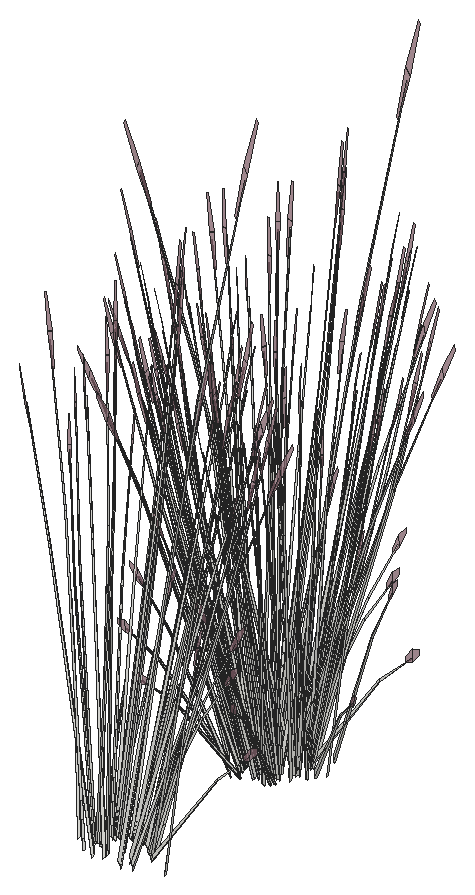
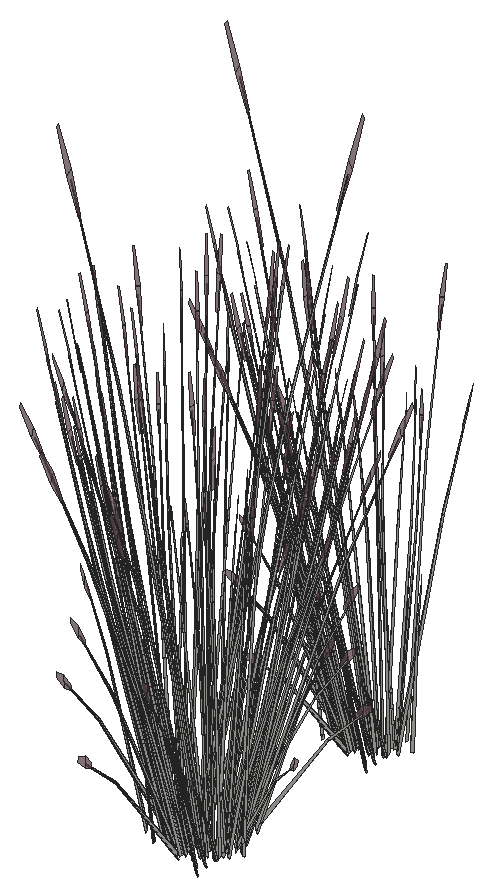
# SketchUp Ruby script. Lengths in inches.
U = 1.inch
M = Sketchup.active_model
def pt(a) = Geom::Point3d.new(a.map { |v| v * U })
def face(e, loops, mat)
  f = e.add_face(loops[0].map { |a| pt(a) })
  loops[1..].each { |l| e.add_face(l.map { |a| pt(a) }).erase! }
  f.material = f.back_material = mat if mat
  f
end
# faces: each face lists its corners as indices into pts; further lists are holes
def faces(e, pts, list, mat = nil) = list.each { |f| face(e, (f[0].is_a?(Array) ? f : [f]).map { |l| l.map { |i| pts[i] } }, mat) }
# xy, xz, yz: faces in a plane at the given z, y or x. An outline is a flat list of corners, or four numbers for a rectangle; further outlines are holes
def ring(l) = l.size == 4 ? [[l[0], l[1]], [l[2], l[1]], [l[2], l[3]], [l[0], l[3]]] : l.each_slice(2).to_a
def flat(e, list, mat, &to3) = list.each { |f| face(e, (f[0].is_a?(Array) ? f : [f]).map { |l| ring(l).map { |u, v| to3.(u, v) } }, mat) }
def xy(e, z, list, mat = nil) = flat(e, list, mat) { |x, y| [x, y, z] }
def xz(e, y, list, mat = nil) = flat(e, list, mat) { |x, z| [x, y, z] }
def yz(e, x, list, mat = nil) = flat(e, list, mat) { |y, z| [x, y, z] }
def lines(e, pts, list) = list.each { |a, b| e.add_line(pt(pts[a]), pt(pts[b])) }
# prism: a flat outline (further loops are holes) pulled along v
def prism(e, loops, v, mat = nil)
  f = face(e, loops, mat); d = Geom::Vector3d.new(v.map { |x| x * U })
  f.pushpull(f.normal.samedirection?(d) ? d.length : -d.length)
end
def box(e, o, s, mat = nil) = prism(e, [[o, [o[0] + s[0], o[1], o[2]], [o[0] + s[0], o[1] + s[1], o[2]], [o[0], o[1] + s[1], o[2]]]], [0, 0, s[2]], mat)
def at(x, y, z, deg = 0) = Geom::Transformation.translation(pt([x, y, z])) * Geom::Transformation.rotation(ORIGIN, Z_AXIS, deg.degrees)
def axes(o, x, y, z) = Geom::Transformation.new([*x, 0, *y, 0, *z, 0, *pt(o).to_a, 1])
def part(name) = M.definitions.add(name)
# library, detail: a bought-in or finely detailed component or shape, given as its bounding box
def library(name, o, s) = part(name).tap { |d| box(d.entities, o, s) }
def detail(e, o, s) = box(e.add_group.entities, o, s)
def put(e, d, t, mat = nil) = e.add_instance(d, t).tap { |i| i.material = mat if mat }
def group(e, t, mat = nil) = e.add_group.tap { |g| g.transformation = t; g.material = mat if mat }.entities
root = M.entities
M.materials.add("LightPink_Translucent").color = [144, 107, 117]
M.materials["LightPink_Translucent"].alpha = 0.75
c1 = part("blade")
p = [[2.15,0.21,22],[0,0.17,0],[0.09,0.45,0],[2.18,0.31,22],[2.29,0.31,22],[0.38,0.45,0],
  [2.48,0.24,33],[2.49,0.24,33],[2.48,0.22,33]]
faces(c1.entities,p,[[0,1,2,3],[4,5,2,3],[6,3,4,7],[8,0,3,6]])
c2 = part("seeds")
p = [[0.3,-0.1,1.38],[-0.01,-0.03,1.59],[-0.01,-0.03,0.03],[0.14,-0.07,-0.07],[0.29,-0.03,3],[0.15,0.01,3.11]]
faces(c2.entities,p,[[0,1,2,3],[1,0,4,5]],"LightPink_Translucent")
c3 = part("blade with seeds")
put(c3.entities,c1,at(0,0,0))
put(c3.entities,c2,axes([2.4,0.25,30.99],[1.5799,-0.05474,1.17369],[-0.12525,1.92788,0.29478],[-0.07173,-0.02425,1.56792]))
put(root,c3,axes([415.32,661.92,154.25],[0.20619,0.42709,-0.10273],[-0.36595,0.20988,-0.57019],[-0.15422,0.05635,0.8664]))
put(root,c3,axes([419.39,663.77,153.32],[-0.07843,-0.39649,-0.0295],[0.37072,-0.09115,-0.13375],[0.07742,0.02514,0.44114]))
put(root,c3,axes([418.43,663.76,154.25],[0.02194,-0.47967,-0.10273],[0.41546,0.01311,-0.57019],[0.16001,0.03332,0.8664]))
put(root,c3,axes([418.79,663.47,153.98],[0.08791,-0.00798,1.47793],[0.24113,-0.36643,-0.23373],[0.15637,0.04837,0.11853]))
put(root,c3,axes([415.19,663.03,154],[-0.28133,-0.19836,0.05432],[0.16379,-0.28248,0.42765],[-0.0902,0.09132,0.65209]))
put(root,c3,axes([415.32,662.51,153.27],[0.14219,-0.09977,1.44779],[0.11971,0.461,0.11706],[-0.22323,0.10419,0.61892]))
put(root,c3,axes([418.45,663.53,154.21],[0.40965,0.01136,-0.60019],[-0.02751,0.47821,0.07243],[0.17355,0.05047,0.84903]))
put(root,c3,axes([414.14,662.8,153.98],[0.0523,0.01265,1.49853],[0.16179,0.41674,-0.1416],[-0.10706,0.10938,0.26519]))
put(root,c3,axes([418.69,663.73,153.82],[0.23317,0.29531,-0.29918],[-0.26625,0.27955,0.38624],[0.13527,0.04253,0.73904]))
put(root,c3,axes([418.57,663.84,154],[-0.02064,0.35866,0.05432],[-0.3116,-0.00983,0.42765],[0.11936,0.03753,0.65209]))
put(root,c3,axes([415.23,663.2,153.82],[-0.35672,0.06741,-0.29918],[-0.09419,-0.38534,0.38624],[-0.10222,0.1035,0.73904]))
put(root,c3,axes([417.86,662.97,153.27],[-0.15222,-0.08126,1.44779],[0.31502,-0.34091,0.11706],[0.19634,0.15379,0.61892]))
put(root,c3,axes([417.88,661.9,153.78],[-0.35411,-0.24507,1.16821],[0.37391,-0.38156,0.50405],[0.11425,0.22994,1.12919]))
put(root,c3,axes([415.33,662.93,154.25],[0.37908,0.26007,-0.10273],[-0.21839,0.37663,-0.57019],[-0.1071,0.13092,0.8664]))
put(root,c3,axes([417.61,664.28,154.25],[0.2442,-0.40372,-0.10273],[0.35364,0.23259,-0.57019],[0.12293,0.11406,0.8664]))
put(root,c3,axes([415.84,662.82,153.27],[0.10236,-0.14492,1.44779],[0.25844,0.39118,0.11706],[-0.17726,0.17814,0.61892]))
put(root,c3,axes([415.52,663.24,153.95],[0.10528,0.43067,-0.43168],[-0.39868,0.07534,-0.33437],[-0.11425,0.11568,0.82598]))
put(root,c3,axes([417.29,664.62,153.98],[0.00121,-0.0571,1.49853],[0.35119,-0.25193,-0.1416],[0.12199,0.08992,0.26519]))
put(root,c3,axes([415.75,663.96,154],[-0.33677,-0.02198,0.05432],[0.00923,-0.33185,0.42765],[-0.03524,0.12712,0.65209]))
put(root,c3,axes([417.9,664.08,153.95],[0.40438,-0.11212,-0.43168],[0.07074,0.4246,-0.33437],[0.10862,0.12168,0.82598]))
put(root,c3,axes([417.7,664.43,154],[-0.18625,0.29962,0.05432],[-0.26523,-0.17444,0.42765],[0.08575,0.09606,0.65209]))
put(root,c3,axes([415.77,663.17,153.27],[0.0763,-0.16212,1.44779],[0.3201,0.3355,0.11706],[-0.1444,0.2091,0.61892]))
put(root,c3,axes([416.66,664.47,154],[-0.30197,0.1603,0.05432],[-0.1478,-0.29231,0.42765],[0.02916,0.12885,0.65209]))
put(root,c3,axes([415.85,664.09,153.82],[-0.27728,0.24833,-0.29918],[-0.26248,-0.28355,0.38624],[-0.03994,0.14407,0.73904]))
put(root,c3,axes([414.9,664.01,153.98],[-0.01019,0.09334,1.47793],[0.28908,0.3247,-0.23373],[-0.07568,0.15355,0.11853]))
put(root,c3,axes([415.82,663.8,154.56],[0.45039,0.02337,-0.11403],[-0.01231,0.44247,-0.63292],[-0.03129,0.17041,0.9617]))
put(root,c3,axes([416.66,664.3,154.25],[0.40102,-0.2196,-0.10273],[0.19707,0.38974,-0.57019],[0.05291,0.16424,0.8664]))
put(root,c3,axes([416.13,663.97,154.23],[0.29336,0.31691,-0.47917],[-0.3099,0.27755,-0.37115],[-0.04464,0.16102,0.91684]))
put(root,c3,axes([417,664.28,153.95],[0.40284,0.11824,-0.43168],[-0.13808,0.40538,-0.33437],[0.03694,0.16321,0.82598]))
put(root,c3,axes([417.23,663.44,153.27],[-0.09368,-0.15143,1.44779],[0.43286,-0.12749,0.11706],[0.09783,0.23774,0.61892]))
put(root,c3,axes([416.82,664.53,153.82],[-0.12355,0.36271,-0.29918],[-0.36044,-0.10579,0.38624],[0.03305,0.14603,0.73904]))
put(root,c3,axes([416.04,663.83,154.51],[-0.01066,0.43628,-0.66621],[-0.44902,-0.0293,0.0804],[-0.04739,0.18483,0.94242]))
put(root,c3,axes([414.87,664.97,153.98],[0.04649,-0.02848,1.49853],[0.38427,0.18941,-0.1416],[-0.00903,0.15771,0.26519]))
put(root,c3,axes([416.46,663.52,153.27],[-0.01003,-0.18103,1.44779],[0.43473,0.12009,0.11706],[-0.02689,0.25798,0.61892]))
put(root,c3,axes([416.85,664.2,154.21],[0.19559,0.38351,-0.60019],[-0.40262,0.21373,0.07243],[0.04574,0.1853,0.84903]))
put(root,c3,axes([416.5625,665.17,153.98],[0.05195,0.07595,1.47793],[0.41921,0.02984,-0.23373],[0.04216,0.1675,0.11853]))
put(root,c3,axes([415.89,664.44,152.84],[0.009,-0.24349,1.30391],[0.40497,0.12861,0.18019],[-0.03509,0.2595,0.61571]))
put(root,c3,axes([416.2,674.35,153.27],[0.09368,0.15143,1.44779],[-0.43286,0.12749,0.11706],[-0.09783,-0.23774,0.61892]))
put(root,c3,axes([416.91,673.35,153.98],[-0.06268,-0.06613,1.47793],[-0.4183,0.04193,-0.23373],[-0.06676,-0.15817,0.11853]))
put(root,c3,axes([417.35,674.47,154.21],[-0.19559,-0.38351,-0.60019],[0.40262,-0.21373,0.07243],[-0.04574,-0.1853,0.84903]))
put(root,c3,axes([418.17,674.84,154.21],[0.01066,-0.43628,-0.60019],[0.44902,0.0293,0.07243],[0.04739,-0.18483,0.84903]))
put(root,c3,axes([418.79,674.16,153.98],[-0.00396,-0.09387,1.47793],[-0.33411,-0.2713,-0.23373],[0.05166,-0.16446,0.11853]))
put(root,c3,axes([417.39,674.14,153.82],[0.12355,-0.36271,-0.29918],[0.36044,0.10579,0.38624],[-0.03305,-0.14603,0.73904]))
put(root,c3,axes([417.66,674.62,153.27],[-0.0763,0.16212,1.44779],[-0.3201,-0.3355,0.11706],[0.1444,-0.2091,0.61892]))
put(root,c3,axes([418.7,673.82,153.98],[-0.04162,0.03603,1.49853],[-0.40776,-0.12155,-0.1416],[-0.01476,-0.15722,0.26519]))
put(root,c3,axes([417.21,674.39,153.95],[-0.40284,-0.11824,-0.43168],[0.13808,-0.40538,-0.33437],[-0.03694,-0.16321,0.82598]))
put(root,c3,axes([418.08,674.7,153.95],[-0.29336,-0.31691,-0.43168],[0.3099,-0.27755,-0.33437],[0.04464,-0.16102,0.82598]))
put(root,c3,axes([416.49,673.13,153.98],[-0.00765,0.05653,1.49853],[-0.37706,0.20517,-0.1416],[-0.11096,-0.10488,0.26519]))
put(root,c3,axes([417.43,674.22,154],[0.4038,0.12331,0.40553],[-0.13808,0.40538,0.33437],[-0.02427,-0.15942,0.83914]))
put(root,c3,axes([417.55,674.37,154.25],[-0.40102,0.2196,-0.10273],[-0.19707,-0.38974,-0.57019],[-0.05291,-0.16424,0.8664]))
put(root,c3,axes([418.38,674.86,154.25],[-0.45039,-0.02337,-0.10273],[0.01231,-0.44247,-0.57019],[0.03129,-0.17041,0.8664]))
put(root,c3,axes([418.35,674.58,153.82],[0.27728,-0.24833,-0.29918],[0.26248,0.28355,0.38624],[0.03994,-0.14407,0.73904]))
put(root,c3,axes([417.54,674.19,154],[0.30197,-0.1603,0.05432],[0.1478,0.29231,0.42765],[-0.02916,-0.12885,0.65209]))
put(root,c3,axes([416.47,674.57,154.21],[-0.34944,-0.22798,-0.60019],[0.24834,-0.39949,0.07243],[-0.1266,-0.13612,0.84903]))
put(root,c3,axes([416.35,674.27,153.82],[-0.06329,-0.37991,-0.29918],[0.36182,-0.10032,0.38624],[-0.09718,-0.10887,0.73904]))
put(root,c3,axes([416.51,674.24,154],[0.18625,-0.29962,0.05432],[0.26523,0.17444,0.42765],[-0.08575,-0.09606,0.65209]))
put(root,c3,axes([415.57,674.83,153.27],[0.15222,0.08126,1.44779],[-0.31502,0.34091,0.11706],[-0.19634,-0.15379,0.61892]))
put(root,c3,axes([416.31,674.59,153.95],[-0.40438,0.11212,-0.43168],[-0.07074,-0.4246,-0.33437],[-0.10862,-0.12168,0.82598]))
put(root,c3,axes([418.35,674.67,154],[0.29182,0.32181,0.40553],[-0.3099,0.27755,0.33437],[0.05383,-0.15098,0.83914]))
put(root,c3,axes([416.59,674.21,154.59],[-0.2735,0.45217,-0.11506],[-0.39608,-0.2605,-0.63862],[-0.13768,-0.12775,0.97037]))
put(root,c3,axes([418.46,674.71,154],[0.33677,0.02198,0.05432],[-0.00923,0.33185,0.42765],[0.03524,-0.12712,0.65209]))
put(root,c3,axes([418.7,675.6,154.21],[0.21406,-0.37215,-0.60019],[0.37511,0.26448,0.07243],[0.12781,-0.13483,0.84903]))
put(root,c3,axes([418.6875,675.43,153.95],[-0.10528,-0.43067,-0.43168],[0.39868,-0.07534,-0.33437],[0.11425,-0.11568,0.82598]))
put(root,c3,axes([415.54,674.08,153.98],[-0.08817,-0.00333,1.47793],[-0.28072,0.33293,-0.23373],[-0.14978,-0.06803,0.11853]))
put(root,c3,axes([418.875,675.73,154.25],[-0.37908,-0.26007,-0.10273],[0.21839,-0.37663,-0.57019],[0.1071,-0.13092,0.8664]))
put(root,c3,axes([417.31,677.15,152.81],[0.35414,0.19019,1.27785],[-0.34693,0.40974,0.50532],[-0.1554,-0.24285,1.07126]))
put(root,c3,axes([419.81,675.62,153.98],[-0.05353,-0.00358,1.49853],[-0.22227,-0.38383,-0.1416],[0.08926,-0.1262,0.26519]))
put(root,c3,axes([418.98,675.47,153.82],[0.35672,-0.06741,-0.29918],[0.09419,0.38534,0.38624],[0.10222,-0.1035,0.73904]))
put(root,c3,axes([415.63,674.83,154],[0.02064,-0.35866,0.05432],[0.3116,0.00983,0.42765],[-0.11936,-0.03753,0.65209]))
put(root,c3,axes([415.51,674.94,153.82],[-0.23317,-0.29531,-0.29918],[0.26625,-0.27955,0.38624],[-0.13527,-0.04253,0.73904]))
put(root,c3,axes([415.76,675.14,154.21],[-0.40965,-0.01136,-0.60019],[0.02751,-0.47821,0.07243],[-0.17355,-0.05047,0.84903]))
put(root,c3,axes([419.01,675.64,154],[0.28133,0.19836,0.05432],[-0.16379,0.28248,0.42765],[0.0902,-0.09132,0.65209]))
put(root,c3,axes([420.01,676.08,153.98],[0.05687,-0.07184,1.47793],[-0.07279,-0.44069,-0.23373],[0.14268,-0.08356,0.11853]))
put(root,c3,axes([415.2,674.36,153.98],[0.03038,0.04707,1.49853],[-0.14646,0.42312,-0.1416],[-0.14833,0.00306,0.26519]))
put(root,c3,axes([415.625,675.23,153.95],[-0.29757,0.31243,-0.43168],[-0.2606,-0.33005,-0.33437],[-0.15119,-0.04754,0.82598]))
put(root,c3,axes([415.78,674.91,154.25],[-0.02194,0.47967,-0.10273],[-0.41546,-0.01311,-0.57019],[-0.16001,-0.03332,0.8664]))
put(root,c3,axes([418.89,676.75,154.25],[-0.20619,-0.42709,-0.10273],[0.36595,-0.20988,-0.57019],[0.15422,-0.05635,0.8664]))
put(root,c3,axes([418.87,676.38,153.95],[0.11102,-0.42903,-0.43168],[0.38064,0.14706,-0.33437],[0.15325,-0.03934,0.82598]))
put(root,c3,axes([415.25,675.57,153.27],[0.16998,-0.01068,1.44779],[-0.11276,0.46299,0.11706],[-0.24224,-0.02864,0.61892]))
put(root,c3,axes([418.8,676.54,154.21],[0.3601,-0.20831,-0.60019],[0.20068,0.4288,0.07243],[0.17399,-0.04871,0.84903]))
put(root,c3,axes([415.15,675.8,154],[-0.15051,-0.3216,0.05432],[0.27447,-0.15741,0.42765],[-0.12099,0.03106,0.65209]))
put(root,c3,axes([419.1,676.58,153.82],[0.34057,0.13158,-0.29918],[-0.09933,0.38387,0.38624],[0.13712,-0.0352,0.73904]))
put(root,c3,axes([415.1,675.97,153.82],[-0.34057,-0.13158,-0.29918],[0.09933,-0.38387,0.38624],[-0.13712,0.0352,0.73904]))
put(root,c3,axes([418.18,676.1,153.27],[-0.16998,0.01068,1.44779],[0.11276,-0.46299,0.11706],[0.24224,0.02864,0.61892]))
put(root,c3,axes([419.05,676.74,154],[0.15051,0.3216,0.05432],[-0.27447,0.15741,0.42765],[0.12099,-0.03106,0.65209]))
put(root,c3,axes([419.03,676.625,154],[-0.11578,0.43006,0.40553],[-0.38064,-0.14706,0.33437],[0.14969,-0.02584,0.83914]))
put(root,c3,axes([416.14,675.9,152.82],[0.11649,-0.06823,1.49584],[0.04017,0.47639,0.11706],[-0.25231,0.06321,0.53462]))
put(root,c3,axes([419.71,678.02,153.98],[-0.03706,-0.04129,1.49853],[0.08106,-0.44261,-0.1416],[0.14596,-0.02828,0.26519]))
put(root,c3,axes([414.89,676.22,153.98],[-0.06692,0.06124,1.47793],[0.00569,0.44742,-0.23373],[-0.15339,0.05818,0.11853]))
put(root,c3,axes([415.34,676.16,153.95],[-0.11102,0.42903,-0.43168],[-0.38064,-0.14706,-0.33437],[-0.15325,0.03934,0.82598]))
put(root,c3,axes([415.32,675.79,154.25],[0.20619,0.42709,-0.10273],[-0.36595,0.20988,-0.57019],[-0.15422,0.05635,0.8664]))
put(root,c3,axes([419.39,677.65,153.32],[-0.07843,-0.39649,-0.0295],[0.37072,-0.09115,-0.13375],[0.07742,0.02514,0.44114]))
put(root,c3,axes([418.43,677.64,154.25],[0.02194,-0.47967,-0.10273],[0.41546,0.01311,-0.57019],[0.16001,0.03332,0.8664]))
put(root,c3,axes([418.79,677.35,153.98],[0.08791,-0.00798,1.47793],[0.24113,-0.36643,-0.23373],[0.15637,0.04837,0.11853]))
put(root,c3,axes([415.27,676.99,154],[-0.10163,-0.43409,0.40553],[0.39868,-0.07534,0.33437],[-0.1175,0.10209,0.83914]))
put(root,c3,axes([415.19,676.91,154],[-0.28133,-0.19836,0.05432],[0.16379,-0.28248,0.42765],[-0.0902,0.09132,0.65209]))
put(root,c3,axes([415.32,676.38,153.27],[0.14219,-0.09977,1.44779],[0.11971,0.461,0.11706],[-0.22323,0.10419,0.61892]))
put(root,c3,axes([418.45,677.41,154.21],[0.40965,0.01136,-0.60019],[-0.02751,0.47821,0.07243],[0.17355,0.05047,0.84903]))
put(root,c3,axes([414.14,676.67,153.98],[0.0523,0.01265,1.49853],[0.16179,0.41674,-0.1416],[-0.10706,0.10938,0.26519]))
put(root,c3,axes([418.69,677.6,153.82],[0.23317,0.29531,-0.29918],[-0.26625,0.27955,0.38624],[0.13527,0.04253,0.73904]))
put(root,c3,axes([418.57,677.72,154],[-0.02064,0.35866,0.05432],[-0.3116,-0.00983,0.42765],[0.11936,0.03753,0.65209]))
put(root,c3,axes([415.23,677.07,153.82],[-0.35672,0.06741,-0.29918],[-0.09419,-0.38534,0.38624],[-0.10222,0.1035,0.73904]))
put(root,c3,axes([418.6,677.6,154],[-0.30217,0.31079,0.40553],[-0.2606,-0.33005,0.33437],[0.14177,0.05733,0.83914]))
put(root,c3,axes([417.86,676.85,153.27],[-0.15222,-0.08126,1.44779],[0.31502,-0.34091,0.11706],[0.19634,0.15379,0.61892]))
put(root,c3,axes([417.88,675.78,153.78],[-0.35411,-0.24507,1.16821],[0.37391,-0.38156,0.50405],[0.11425,0.22994,1.12919]))
put(root,c3,axes([415.33,676.81,154.25],[0.37908,0.26007,-0.10273],[-0.21839,0.37663,-0.57019],[-0.1071,0.13092,0.8664]))
put(root,c3,axes([417.61,678.16,154.25],[0.2442,-0.40372,-0.10273],[0.35364,0.23259,-0.57019],[0.12293,0.11406,0.8664]))
put(root,c3,axes([415.84,676.69,153.27],[0.10236,-0.14492,1.44779],[0.25844,0.39118,0.11706],[-0.17726,0.17814,0.61892]))
put(root,c3,axes([415.52,677.12,153.95],[0.10528,0.43067,-0.43168],[-0.39868,0.07534,-0.33437],[-0.11425,0.11568,0.82598]))
put(root,c3,axes([417.29,678.49,153.98],[0.00121,-0.0571,1.49853],[0.35119,-0.25193,-0.1416],[0.12199,0.08992,0.26519]))
put(root,c3,axes([415.75,677.84,154],[-0.33677,-0.02198,0.05432],[0.00923,-0.33185,0.42765],[-0.03524,0.12712,0.65209]))
put(root,c3,axes([415.85,677.87,154],[-0.29182,-0.32181,0.40553],[0.3099,-0.27755,0.33437],[-0.05383,0.15098,0.83914]))
put(root,c3,axes([417.9,677.96,153.95],[0.40438,-0.11212,-0.43168],[0.07074,0.4246,-0.33437],[0.10862,0.12168,0.82598]))
put(root,c3,axes([417.7,678.31,154],[-0.18625,0.29962,0.05432],[-0.26523,-0.17444,0.42765],[0.08575,0.09606,0.65209]))
put(root,c3,axes([415.77,677.05,153.27],[0.0763,-0.16212,1.44779],[0.3201,0.3355,0.11706],[-0.1444,0.2091,0.61892]))
put(root,c3,axes([416.66,678.35,154],[-0.30197,0.1603,0.05432],[-0.1478,-0.29231,0.42765],[0.02916,0.12885,0.65209]))
put(root,c3,axes([415.85,677.96,153.82],[-0.27728,0.24833,-0.29918],[-0.26248,-0.28355,0.38624],[-0.03994,0.14407,0.73904]))
put(root,c3,axes([414.9,677.89,153.98],[-0.01019,0.09334,1.47793],[0.28908,0.3247,-0.23373],[-0.07568,0.15355,0.11853]))
put(root,c3,axes([415.82,677.68,154.56],[0.45039,0.02337,-0.11403],[-0.01231,0.44247,-0.63292],[-0.03129,0.17041,0.9617]))
put(root,c3,axes([416.66,678.17,154.25],[0.40102,-0.2196,-0.10273],[0.19707,0.38974,-0.57019],[0.05291,0.16424,0.8664]))
put(root,c3,axes([416.13,677.85,154.23],[0.29336,0.31691,-0.47917],[-0.3099,0.27755,-0.37115],[-0.04464,0.16102,0.91684]))
put(root,c3,axes([417,678.15,153.95],[0.40284,0.11824,-0.43168],[-0.13808,0.40538,-0.33437],[0.03694,0.16321,0.82598]))
put(root,c3,axes([417.23,677.32,153.27],[-0.09368,-0.15143,1.44779],[0.43286,-0.12749,0.11706],[0.09783,0.23774,0.61892]))
put(root,c3,axes([416.82,678.4,153.82],[-0.12355,0.36271,-0.29918],[-0.36044,-0.10579,0.38624],[0.03305,0.14603,0.73904]))
put(root,c3,axes([416.04,677.7,154.51],[-0.01066,0.43628,-0.66621],[-0.44902,-0.0293,0.0804],[-0.04739,0.18483,0.94242]))
put(root,c3,axes([414.87,678.85,153.98],[0.04649,-0.02848,1.49853],[0.38427,0.18941,-0.1416],[-0.00903,0.15771,0.26519]))
put(root,c3,axes([416.46,677.39,153.27],[-0.01003,-0.18103,1.44779],[0.43473,0.12009,0.11706],[-0.02689,0.25798,0.61892]))
put(root,c3,axes([416.85,678.08,154.21],[0.19559,0.38351,-0.60019],[-0.40262,0.21373,0.07243],[0.04574,0.1853,0.84903]))
put(root,c3,axes([416.5625,679.05,153.98],[0.05195,0.07595,1.47793],[0.41921,0.02984,-0.23373],[0.04216,0.1675,0.11853]))
put(root,c3,axes([415.89,678.32,152.84],[0.009,-0.24349,1.30391],[0.40497,0.12861,0.18019],[-0.03509,0.2595,0.61571]))
